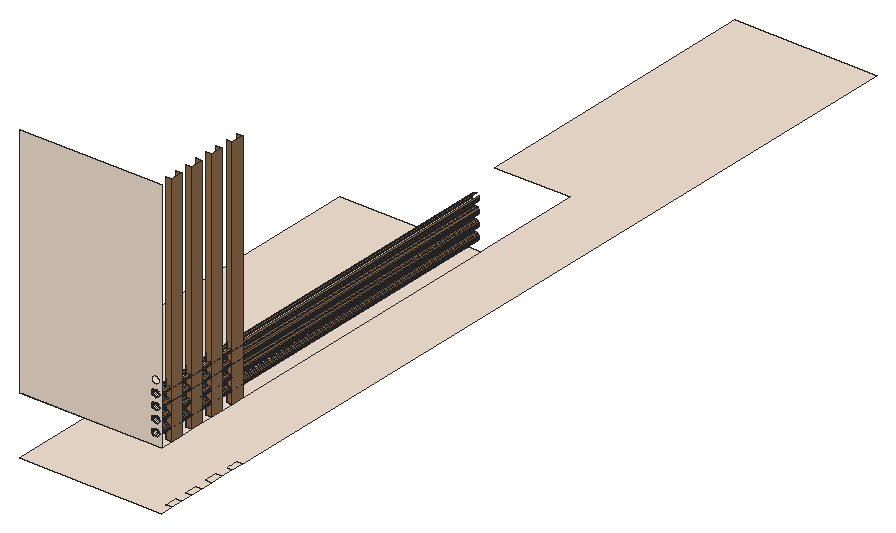
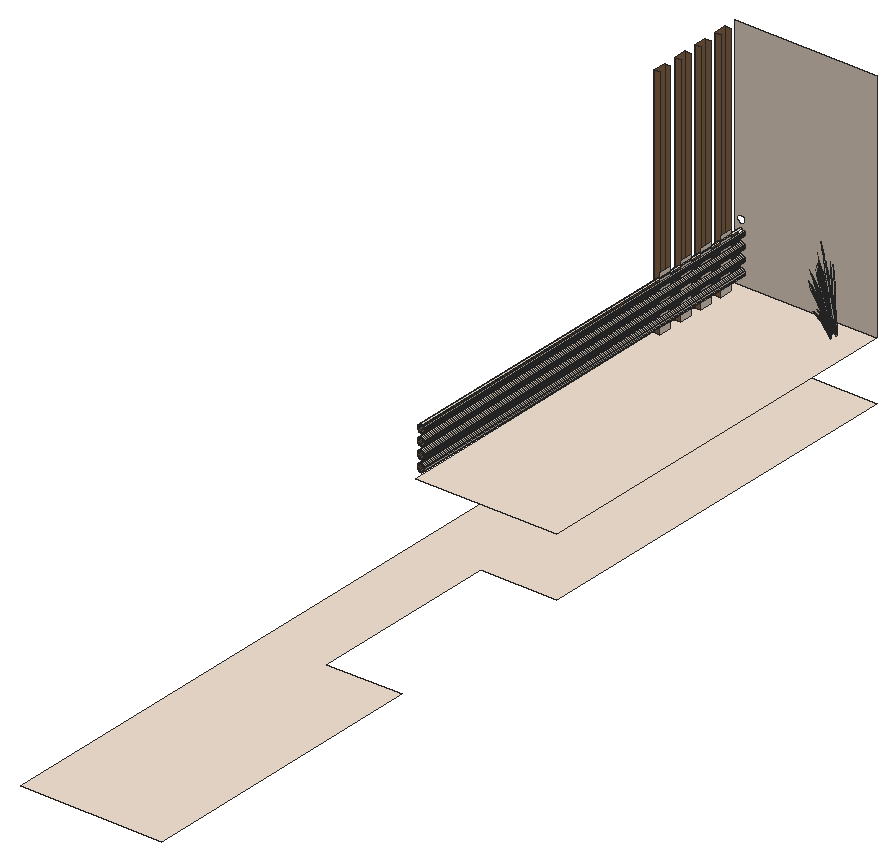
# SketchUp Ruby script. Lengths in inches.
U = 1.inch
M = Sketchup.active_model
def pt(a) = Geom::Point3d.new(a.map { |v| v * U })
def face(e, loops, mat)
  f = e.add_face(loops[0].map { |a| pt(a) })
  loops[1..].each { |l| e.add_face(l.map { |a| pt(a) }).erase! }
  f.material = f.back_material = mat if mat
  f
end
# faces: each face lists its corners as indices into pts; further lists are holes
def faces(e, pts, list, mat = nil) = list.each { |f| face(e, (f[0].is_a?(Array) ? f : [f]).map { |l| l.map { |i| pts[i] } }, mat) }
# xy, xz, yz: faces in a plane at the given z, y or x. An outline is a flat list of corners, or four numbers for a rectangle; further outlines are holes
def ring(l) = l.size == 4 ? [[l[0], l[1]], [l[2], l[1]], [l[2], l[3]], [l[0], l[3]]] : l.each_slice(2).to_a
def flat(e, list, mat, &to3) = list.each { |f| face(e, (f[0].is_a?(Array) ? f : [f]).map { |l| ring(l).map { |u, v| to3.(u, v) } }, mat) }
def xy(e, z, list, mat = nil) = flat(e, list, mat) { |x, y| [x, y, z] }
def xz(e, y, list, mat = nil) = flat(e, list, mat) { |x, z| [x, y, z] }
def yz(e, x, list, mat = nil) = flat(e, list, mat) { |y, z| [x, y, z] }
def lines(e, pts, list) = list.each { |a, b| e.add_line(pt(pts[a]), pt(pts[b])) }
# prism: a flat outline (further loops are holes) pulled along v
def prism(e, loops, v, mat = nil)
  f = face(e, loops, mat); d = Geom::Vector3d.new(v.map { |x| x * U })
  f.pushpull(f.normal.samedirection?(d) ? d.length : -d.length)
end
def box(e, o, s, mat = nil) = prism(e, [[o, [o[0] + s[0], o[1], o[2]], [o[0] + s[0], o[1] + s[1], o[2]], [o[0], o[1] + s[1], o[2]]]], [0, 0, s[2]], mat)
def at(x, y, z, deg = 0) = Geom::Transformation.translation(pt([x, y, z])) * Geom::Transformation.rotation(ORIGIN, Z_AXIS, deg.degrees)
def axes(o, x, y, z) = Geom::Transformation.new([*x, 0, *y, 0, *z, 0, *pt(o).to_a, 1])
def part(name) = M.definitions.add(name)
# library, detail: a bought-in or finely detailed component or shape, given as its bounding box
def library(name, o, s) = part(name).tap { |d| box(d.entities, o, s) }
def detail(e, o, s) = box(e.add_group.entities, o, s)
def put(e, d, t, mat = nil) = e.add_instance(d, t).tap { |i| i.material = mat if mat }
def group(e, t, mat = nil) = e.add_group.tap { |g| g.transformation = t; g.material = mat if mat }.entities
root = M.entities
M.materials.add("C01_Vanilla_Cream").color = [244, 228, 212]
M.materials.add("LightPink_Translucent").color = [144, 107, 117]
M.materials["LightPink_Translucent"].alpha = 0.75
M.materials.add("Wood_Floor_01_1K").color = [146, 111, 76]
c1 = part("blade")
p = [[2.15,0.21,22],[0,0.17,0],[0.09,0.45,0],[2.18,0.31,22],[2.29,0.31,22],[0.38,0.45,0],
  [2.48,0.24,33],[2.49,0.24,33],[2.48,0.22,33]]
faces(c1.entities,p,[[0,1,2,3],[4,5,2,3],[6,3,4,7],[8,0,3,6]])
c2 = part("seeds")
p = [[0.3,-0.1,1.38],[-0.01,-0.03,1.59],[-0.01,-0.03,0.03],[0.14,-0.07,-0.07],[0.29,-0.03,3],[0.15,0.01,3.11]]
faces(c2.entities,p,[[0,1,2,3],[1,0,4,5]],"LightPink_Translucent")
c3 = part("blade with seeds")
put(c3.entities,c1,at(0,0,0))
put(c3.entities,c2,axes([2.4,0.25,30.99],[1.5799,-0.05474,1.17369],[-0.12525,1.92788,0.29478],[-0.07173,-0.02425,1.56792]))
xy(root,282,[[288,12,288,216,326.85,216,326.85,314.71,288,314.71,288,468,360,468,360,63.65,357,63.65,357,57.2,360,57.2,360,50.74,357,50.74,357,44.28,360,44.28,360,37.83,357,37.83,357,31.37,360,31.37,360,24.91,357,24.91,357,18.46,360,18.46,360,12],[357,18.46,360,24.91],[357,31.37,360,37.83],[357,44.28,360,50.74],[357,57.2,360,63.65]],"C01_Vanilla_Cream")
xy(root,312,[[288,12,360,12,360,18.46,357,18.46,357,24.91,360,24.91,360,31.37,357,31.37,357,37.83,360,37.83,360,44.28,357,44.28,357,50.74,360,50.74,360,57.2,357,57.2,357,63.65,360,63.65,360,216,288,216],[357,18.46,360,24.91],[357,31.37,360,37.83],[357,44.28,360,50.74],[357,57.2,360,63.65]],"C01_Vanilla_Cream")
xz(root,12,[[[288,312,360,432],[357,334,357.52,334.07,358,334.27,358.41,334.59,358.73,335,358.93,335.48,359,336,358.93,336.52,358.73,337,358.41,337.41,358,337.73,357.52,337.93,357,338,356.48,337.93,356,337.73,355.59,337.41,355.27,337,355.07,336.52,355,336,355.07,335.48,355.27,335,355.59,334.59,356,334.27,356.48,334.07],[357,340,357.52,340.07,358,340.27,358.41,340.59,358.73,341,358.93,341.48,359,342,358.93,342.52,358.73,343,358.41,343.41,358,343.73,357.52,343.93,357,344,356.48,343.93,356,343.73,355.59,343.41,355.27,343,355.07,342.52,355,342,355.07,341.48,355.27,341,355.59,340.59,356,340.27,356.48,340.07],[357,328,357.52,328.07,358,328.27,358.41,328.59,358.73,329,358.93,329.48,359,330,358.93,330.52,358.73,331,358.41,331.41,358,331.73,357.52,331.93,357,332,356.48,331.93,356,331.73,355.59,331.41,355.27,331,355.07,330.52,355,330,355.07,329.48,355.27,329,355.59,328.59,356,328.27,356.48,328.07],[357,322,357.52,322.07,358,322.27,358.41,322.59,358.73,323,358.93,323.48,359,324,358.93,324.52,358.73,325,358.41,325.41,358,325.73,357.52,325.93,357,326,356.48,325.93,356,325.73,355.59,325.41,355.27,325,355.07,324.52,355,324,355.07,323.48,355.27,323,355.59,322.59,356,322.27,356.48,322.07],[357,316,357.52,316.07,358,316.27,358.41,316.59,358.73,317,358.93,317.48,359,318,358.93,318.52,358.73,319,358.41,319.41,358,319.73,357.52,319.93,357,320,356.48,319.93,356,319.73,355.59,319.41,355.27,319,355.07,318.52,355,318,355.07,317.48,355.27,317,355.59,316.59,356,316.27,356.48,316.07]]],"C01_Vanilla_Cream")
xz(root,18.46,[[357,312,360,432]],"Wood_Floor_01_1K")
xz(root,24.91,[[357,312,360,432]],"Wood_Floor_01_1K")
xz(root,31.37,[[357,312,360,432]],"Wood_Floor_01_1K")
xz(root,37.83,[[357,312,360,432]],"Wood_Floor_01_1K")
xz(root,44.28,[[357,312,360,432]],"Wood_Floor_01_1K")
xz(root,50.74,[[357,312,360,432]],"Wood_Floor_01_1K")
xz(root,57.2,[[357,312,360,432]],"Wood_Floor_01_1K")
xz(root,63.65,[[357,312,360,432]],"Wood_Floor_01_1K")
yz(root,357,[[18.46,312,24.91,316],[31.37,312,37.83,316],[44.28,312,50.74,316],[57.2,312,63.65,316],[18.46,316,24.91,320],
  [31.37,316,37.83,320],[44.28,316,50.74,320],[57.2,316,63.65,320],[18.46,320,24.91,322],[31.37,320,37.83,322],
  [44.28,320,50.74,322],[57.2,320,63.65,322],[18.46,322,24.91,326],[31.37,322,37.83,326],[44.28,322,50.74,326],
  [57.2,322,63.65,326],[18.46,326,24.91,328],[31.37,326,37.83,328],[44.28,326,50.74,328],[57.2,326,63.65,328],
  [18.46,328,24.91,332],[31.37,328,37.83,332],[44.28,328,50.74,332],[57.2,328,63.65,332],[18.46,332,24.91,334],
  [31.37,332,37.83,334],[44.28,332,50.74,334],[57.2,332,63.65,334],[18.46,334,24.91,338],[31.37,334,37.83,338],
  [44.28,334,50.74,338],[57.2,334,63.65,338],[18.46,338,24.91,340],[31.37,338,37.83,340],[44.28,338,50.74,340],
  [57.2,338,63.65,340]],"C01_Vanilla_Cream")
yz(root,360,[[18.46,312,24.91,432],[31.37,312,37.83,432],[44.28,312,50.74,432],[57.2,312,63.65,432]],"Wood_Floor_01_1K")
p = [[356.48,216,316.07],[357,216,316],[357,63.65,316],[357,57.2,316],[357,50.74,316],[357,44.28,316],
  [357,37.83,316],[357,31.37,316],[357,24.91,316],[357,18.46,316],[357,12,316],[356.48,12,316.07],
  [357.52,216,316.07],[357.52,12,316.07],[356,216,316.27],[356,12,316.27],[358,216,316.27],[358,12,316.27],
  [355.59,216,316.59],[355.59,12,316.59],[358.41,216,316.59],[358.41,12,316.59],[355.27,216,317],[355.27,12,317],
  [358.73,216,317],[358.73,12,317],[355.07,216,317.48],[355.07,12,317.48],[358.93,216,317.48],[358.93,12,317.48],
  [355,216,318],[355,12,318],[359,216,318],[359,12,318],[355.07,216,318.52],[355.07,12,318.52],
  [358.93,216,318.52],[358.93,12,318.52],[355.27,216,319],[355.27,12,319],[358.73,216,319],[358.73,12,319],
  [355.59,216,319.41],[355.59,12,319.41],[358.41,216,319.41],[358.41,12,319.41],[356,216,319.73],[356,12,319.73],
  [358,216,319.73],[358,12,319.73],[356.48,216,319.93],[356.48,12,319.93],[357.52,216,319.93],[357.52,12,319.93],
  [357,216,320],[357,12,320],[357,18.46,320],[357,24.91,320],[357,31.37,320],[357,37.83,320],
  [357,44.28,320],[357,50.74,320],[357,57.2,320],[357,63.65,320],[356.48,216,322.07],[357,216,322],
  [357,63.65,322],[357,57.2,322],[357,50.74,322],[357,44.28,322],[357,37.83,322],[357,31.37,322],
  [357,24.91,322],[357,18.46,322],[357,12,322],[356.48,12,322.07],[357.52,216,322.07],[357.52,12,322.07],
  [356,216,322.27],[356,12,322.27],[358,216,322.27],[358,12,322.27],[355.59,216,322.59],[355.59,12,322.59],
  [358.41,216,322.59],[358.41,12,322.59],[355.27,216,323],[355.27,12,323],[358.73,216,323],[358.73,12,323],
  [355.07,216,323.48],[355.07,12,323.48],[358.93,216,323.48],[358.93,12,323.48],[355,216,324],[355,12,324],
  [359,216,324],[359,12,324],[355.07,216,324.52],[355.07,12,324.52],[358.93,216,324.52],[358.93,12,324.52],
  [355.27,216,325],[355.27,12,325],[358.73,216,325],[358.73,12,325],[355.59,216,325.41],[355.59,12,325.41],
  [358.41,216,325.41],[358.41,12,325.41],[356,216,325.73],[356,12,325.73],[358,216,325.73],[358,12,325.73],
  [356.48,216,325.93],[356.48,12,325.93],[357.52,216,325.93],[357.52,12,325.93],[357,216,326],[357,12,326],
  [357,18.46,326],[357,24.91,326],[357,31.37,326],[357,37.83,326],[357,44.28,326],[357,50.74,326],
  [357,57.2,326],[357,63.65,326],[356.48,216,328.07],[357,216,328],[357,63.65,328],[357,57.2,328],
  [357,50.74,328],[357,44.28,328],[357,37.83,328],[357,31.37,328],[357,24.91,328],[357,18.46,328],
  [357,12,328],[356.48,12,328.07],[357.52,216,328.07],[357.52,12,328.07],[356,216,328.27],[356,12,328.27],
  [358,216,328.27],[358,12,328.27],[355.59,216,328.59],[355.59,12,328.59],[358.41,216,328.59],[358.41,12,328.59],
  [355.27,216,329],[355.27,12,329],[358.73,216,329],[358.73,12,329],[355.07,216,329.48],[355.07,12,329.48],
  [358.93,216,329.48],[358.93,12,329.48],[355,216,330],[355,12,330],[359,216,330],[359,12,330],
  [355.07,216,330.52],[355.07,12,330.52],[358.93,216,330.52],[358.93,12,330.52],[355.27,216,331],[355.27,12,331],
  [358.73,216,331],[358.73,12,331],[355.59,216,331.41],[355.59,12,331.41],[358.41,216,331.41],[358.41,12,331.41],
  [356,216,331.73],[356,12,331.73],[358,216,331.73],[358,12,331.73],[356.48,216,331.93],[356.48,12,331.93],
  [357.52,216,331.93],[357.52,12,331.93],[357,216,332],[357,12,332],[357,18.46,332],[357,24.91,332],
  [357,31.37,332],[357,37.83,332],[357,44.28,332],[357,50.74,332],[357,57.2,332],[357,63.65,332],
  [356.48,216,334.07],[357,216,334],[357,63.65,334],[357,57.2,334],[357,50.74,334],[357,44.28,334],
  [357,37.83,334],[357,31.37,334],[357,24.91,334],[357,18.46,334],[357,12,334],[356.48,12,334.07],
  [357.52,216,334.07],[357.52,12,334.07],[356,216,334.27],[356,12,334.27],[358,216,334.27],[358,12,334.27],
  [355.59,216,334.59],[355.59,12,334.59],[358.41,216,334.59],[358.41,12,334.59],[355.27,216,335],[355.27,12,335],
  [358.73,216,335],[358.73,12,335],[355.07,216,335.48],[355.07,12,335.48],[358.93,216,335.48],[358.93,12,335.48],
  [355,216,336],[355,12,336],[359,216,336],[359,12,336],[355.07,216,336.52],[355.07,12,336.52],
  [358.93,216,336.52],[358.93,12,336.52],[355.27,216,337],[355.27,12,337],[358.73,216,337],[358.73,12,337],
  [355.59,216,337.41],[355.59,12,337.41],[357,216,338],[356.48,216,337.93],[356.48,12,337.93],[357,12,338],
  [357,18.46,338],[357,24.91,338],[357,31.37,338],[357,37.83,338],[357,44.28,338],[357,50.74,338],
  [357,57.2,338],[357,63.65,338],[357.52,216,337.93],[357.52,12,337.93]]
faces(root,p,[[0,1,2,3,4,5,6,7,8,9,10,11],[14,0,11,15],[18,14,15,19],[22,18,19,23],[26,22,23,27],[30,26,27,31],[34,30,31,35],[38,34,35,39],
  [42,38,39,43],[46,42,43,47],[50,46,47,51],[54,50,51,55,56,57,58,59,60,61,62,63],[64,65,66,67,68,69,70,71,72,73,74,75],[78,64,75,79],[82,78,79,83],[86,82,83,87],
  [90,86,87,91],[94,90,91,95],[98,94,95,99],[102,98,99,103],[106,102,103,107],[110,106,107,111],[114,110,111,115],[118,114,115,119,120,121,122,123,124,125,126,127],
  [128,129,130,131,132,133,134,135,136,137,138,139],[142,128,139,143],[146,142,143,147],[150,146,147,151],[154,150,151,155],[158,154,155,159],[162,158,159,163],[166,162,163,167],
  [170,166,167,171],[174,170,171,175],[178,174,175,179],[182,178,179,183,184,185,186,187,188,189,190,191],[192,193,194,195,196,197,198,199,200,201,202,203],[206,192,203,207],[210,206,207,211],[214,210,211,215],
  [218,214,215,219],[222,218,219,223],[226,222,223,227],[230,226,227,231],[234,230,231,235],[236,237,238,239,240,241,242,243,244,245,246,247]],"C01_Vanilla_Cream")
faces(root,p,[[1,12,13,10,9,8,7,6,5,4,3,2],[12,16,17,13],[16,20,21,17],[20,24,25,21],[24,28,29,25],[28,32,33,29],[32,36,37,33],[36,40,41,37],
  [40,44,45,41],[44,48,49,45],[48,52,53,49],[52,54,63,62,61,60,59,58,57,56,55,53],[65,76,77,74,73,72,71,70,69,68,67,66],[76,80,81,77],[80,84,85,81],[84,88,89,85],
  [88,92,93,89],[92,96,97,93],[96,100,101,97],[100,104,105,101],[104,108,109,105],[108,112,113,109],[112,116,117,113],[116,118,127,126,125,124,123,122,121,120,119,117],
  [129,140,141,138,137,136,135,134,133,132,131,130],[140,144,145,141],[144,148,149,145],[148,152,153,149],[152,156,157,153],[156,160,161,157],[160,164,165,161],[164,168,169,165],
  [168,172,173,169],[172,176,177,173],[176,180,181,177],[180,182,191,190,189,188,187,186,185,184,183,181],[193,204,205,202,201,200,199,198,197,196,195,194],[204,208,209,205],[208,212,213,209],[212,216,217,213],
  [216,220,221,217],[220,224,225,221],[224,228,229,225],[228,232,233,229],[248,236,247,246,245,244,243,242,241,240,239,249]],"Wood_Floor_01_1K")
put(root,c3,axes([300.94,21.08,313.12],[-0.08333,-0.03881,1.32257],[-0.21404,-0.4336,-0.20205],[0.14439,-0.11767,0.22528]))
put(root,c3,axes([300.48,24.23,315.79],[-0.31678,-0.30846,0.2656],[0.36171,-0.29199,-0.3429],[0.18378,0.04443,0.65611]))
put(root,c3,axes([300.67,21.59,313.51],[0.52105,0.24633,-0.37238],[-0.31144,0.44171,0],[0.11867,0.0561,1.18128]))
put(root,c3,axes([300.77,24.51,315.55],[-0.02803,0.37463,0.04823],[-0.42332,-0.01027,0.37966],[0.16216,0.0392,0.57892]))
put(root,c3,axes([300.65,25.09,313.12],[0.04056,-0.07113,1.32257],[0.51066,-0.20948,-0.20205],[0.15482,0.10842,0.22528]))
put(root,c3,axes([300.81,24.39,315.55],[-0.41051,0.32462,0.36002],[-0.35404,-0.34474,0.29685],[0.1926,0.05988,0.74497]))
put(root,c3,axes([300.92,22.12,315.51],[-0.14302,-0.44985,-0.38324],[0.54163,-0.07869,-0.29685],[0.15522,-0.12083,0.7333]))
put(root,c3,axes([301.875,24.44,314.95],[-0.10656,-0.41414,-0.02619],[0.50364,-0.09521,-0.11874],[0.10517,0.02626,0.39164]))
put(root,c3,axes([301.01,23.37,315.79],[-0.46269,-0.13744,0.2656],[0.13495,-0.40096,-0.3429],[0.18628,-0.03677,0.65611]))
put(root,c3,axes([299.92,22.53,313.54],[0.57914,0.08077,-0.46765],[-0.12221,0.49823,-0.12274],[0.17283,0.06037,1.03225]))
put(root,c3,axes([302.38,22.83,313.7],[-0.34516,-0.31503,-0.04866],[0.37803,-0.28865,-0.22062],[0.10711,-0.02032,0.72768]))
put(root,c3,axes([301.59,21.22,314.07],[-0.18544,0.25079,0.86145],[-0.15939,-0.33694,0.63294],[0.15316,-0.08443,0.18974]))
put(root,c3,axes([301.37,22.34,315.55],[0.3822,0.20719,0.04823],[-0.22252,0.29505,0.37966],[0.12254,-0.09539,0.57892]))
put(root,c3,axes([301.26,22.25,315.55],[0.13808,0.45342,0.36002],[-0.54163,0.07869,0.29685],[0.15963,-0.10664,0.74497]))
put(root,c3,axes([299.8,23.6,314.91],[-0.2068,-0.08488,1.28532],[0.42797,-0.35609,0.10393],[0.26673,0.16064,0.54946]))
put(root,c3,axes([302.45,22.32,315.53],[-0.07272,-0.00374,1.33037],[-0.30197,-0.40092,-0.12571],[0.12127,-0.13182,0.23543]))
put(root,c3,axes([301.32,22.17,315.39],[0.48462,-0.07041,-0.2656],[0.12797,0.4025,0.3429],[0.13888,-0.10811,0.65611]))
put(root,c3,axes([300.9375,22.3,315.74],[0.29081,-0.38873,-0.53284],[0.5096,0.27626,0.0643],[0.17364,-0.14084,0.75375]))
put(root,c3,axes([301.42,23.49,315.55],[0.20448,0.33592,0.04823],[-0.37288,0.16442,0.37966],[0.16437,-0.03244,0.57892]))
put(root,c3,axes([300.93,24.39,315.39],[0.31678,0.30846,-0.2656],[-0.36171,0.29199,0.3429],[0.18378,0.04443,0.65611]))
put(root,c3,axes([300.57,24.43,315.78],[0.02981,-0.50103,-0.0912],[0.56442,0.01369,-0.50621],[0.21738,0.0348,0.76918]))
put(root,c3,axes([301.2,23.5,315.78],[-0.28012,-0.44611,-0.0912],[0.49717,-0.21923,-0.50621],[0.20951,-0.05886,0.76918]))
put(root,c3,axes([301.39,23.37,315.55],[-0.15729,0.44921,0.36002],[-0.51712,-0.15361,0.29685],[0.20336,-0.027,0.74497]))
put(root,c3,axes([301.0625,24.125,315.54],[0.11943,-0.00833,1.31208],[0.32759,-0.38275,-0.2075],[0.21244,0.05052,0.10523]))
put(root,c3,axes([301.18,23.12,315.51],[0.15083,-0.44814,-0.38324],[0.51712,0.15361,-0.29685],[0.2082,-0.04109,0.7333]))
put(root,c3,axes([302.47,23.4,314.07],[-0.34399,0.08133,0.86145],[0.16192,-0.33614,0.63294],[0.18249,0.023,0.18974]))
put(root,c3,axes([301.36,21.94,313.94],[-0.19889,-0.01459,1.07251],[-0.20376,-0.39145,-0.23066],[0.24434,-0.11074,0.45856]))
put(root,c3,axes([301.49,23.32,315.39],[0.46269,0.13744,-0.2656],[-0.13495,0.40096,0.3429],[0.18628,-0.03677,0.65611]))
put(root,c3,axes([300.6,24.1875,315.74],[0.55654,0.01186,-0.53284],[-0.03738,0.49951,0.0643],[0.23578,0.05271,0.75375]))
put(root,c3,axes([301.73,23.24,313.49],[-0.35858,0.05912,1.06187],[-0.05708,-0.47061,0.06078],[0.25115,-0.07123,0.60425]))
put(root,c3,axes([302.12,22.9375,313.12],[-0.0291,-0.0748,1.32257],[0.20181,-0.43752,-0.20205],[0.20357,-0.00629,0.22528]))
put(root,c3,axes([302.3125,24.83,315.53],[-0.05034,-0.04313,1.33037],[0.11012,-0.46232,-0.12571],[0.1983,-0.02954,0.23543]))
put(root,c3,axes([300.23,22.83,314.91],[-0.23093,0.01116,1.28532],[0.15319,-0.4836,0.10393],[0.32909,0.02991,0.54946]))
put(root,c3,axes([301.08,23.28,315.74],[0.48922,-0.21758,-0.53284],[0.27264,0.44789,0.0643],[0.23638,-0.05088,0.75375]))
put(root,c3,axes([302.72,22.8,315.54],[0.07726,-0.07504,1.31208],[-0.09888,-0.46032,-0.2075],[0.19384,-0.08728,0.10523]))
put(root,c3,axes([301.83,23.94,313.94],[-0.13408,-0.12117,1.07251],[0.17446,-0.40083,-0.23066],[0.27128,0.0543,0.45856]))
